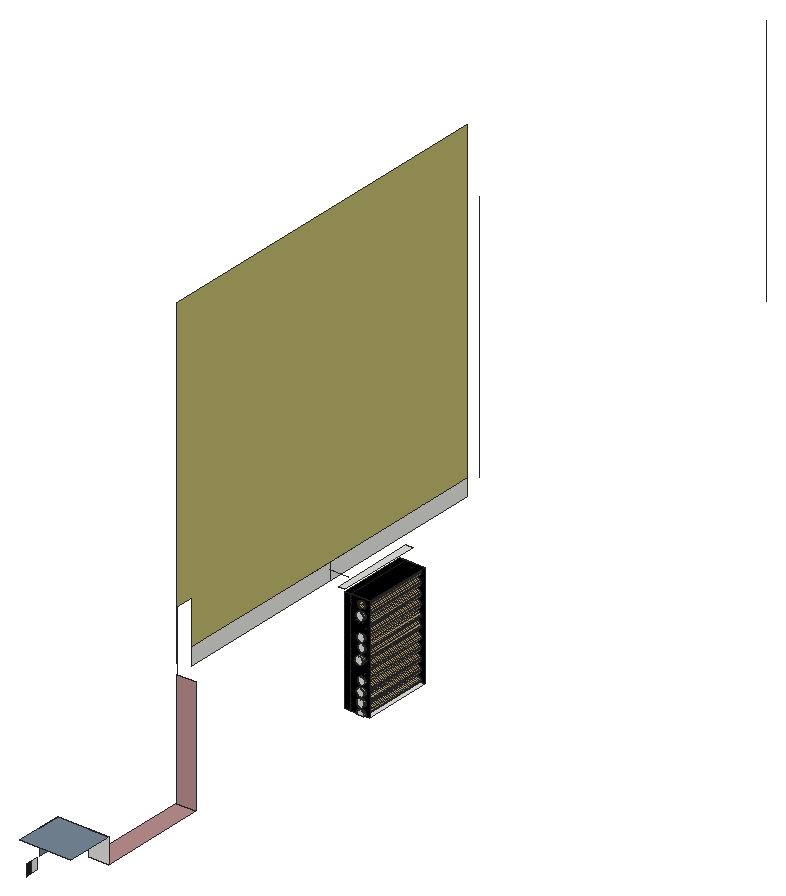
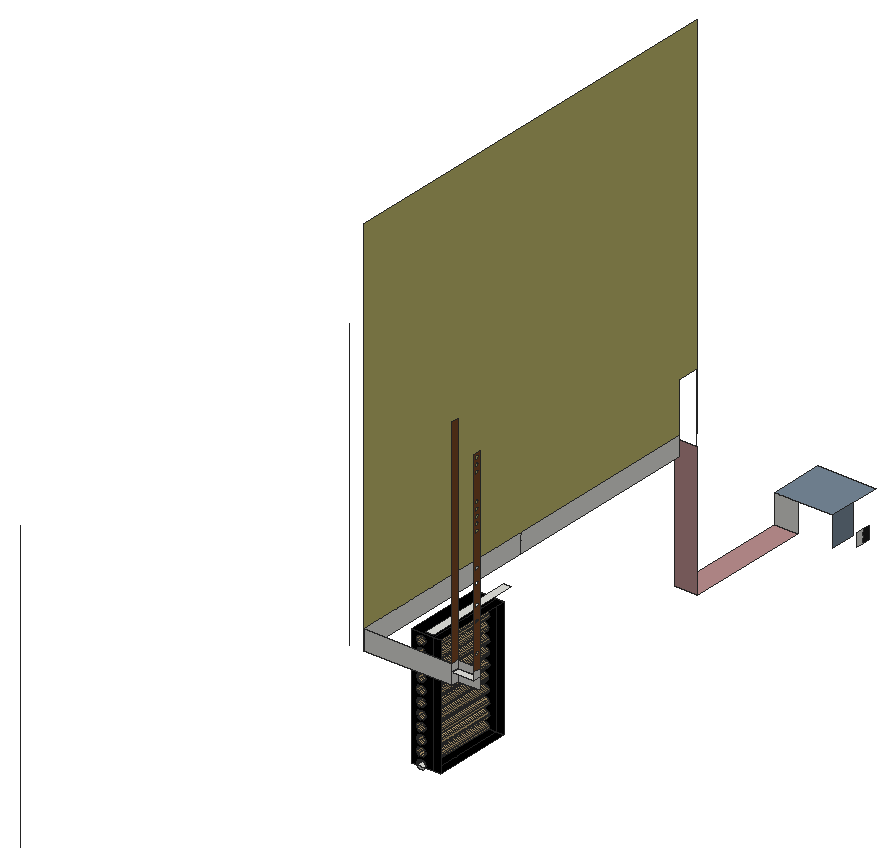
# SketchUp Ruby script. Lengths in inches.
U = 1.inch
M = Sketchup.active_model
def pt(a) = Geom::Point3d.new(a.map { |v| v * U })
def face(e, loops, mat)
  f = e.add_face(loops[0].map { |a| pt(a) })
  loops[1..].each { |l| e.add_face(l.map { |a| pt(a) }).erase! }
  f.material = f.back_material = mat if mat
  f
end
# faces: each face lists its corners as indices into pts; further lists are holes
def faces(e, pts, list, mat = nil) = list.each { |f| face(e, (f[0].is_a?(Array) ? f : [f]).map { |l| l.map { |i| pts[i] } }, mat) }
# xy, xz, yz: faces in a plane at the given z, y or x. An outline is a flat list of corners, or four numbers for a rectangle; further outlines are holes
def ring(l) = l.size == 4 ? [[l[0], l[1]], [l[2], l[1]], [l[2], l[3]], [l[0], l[3]]] : l.each_slice(2).to_a
def flat(e, list, mat, &to3) = list.each { |f| face(e, (f[0].is_a?(Array) ? f : [f]).map { |l| ring(l).map { |u, v| to3.(u, v) } }, mat) }
def xy(e, z, list, mat = nil) = flat(e, list, mat) { |x, y| [x, y, z] }
def xz(e, y, list, mat = nil) = flat(e, list, mat) { |x, z| [x, y, z] }
def yz(e, x, list, mat = nil) = flat(e, list, mat) { |y, z| [x, y, z] }
def lines(e, pts, list) = list.each { |a, b| e.add_line(pt(pts[a]), pt(pts[b])) }
# prism: a flat outline (further loops are holes) pulled along v
def prism(e, loops, v, mat = nil)
  f = face(e, loops, mat); d = Geom::Vector3d.new(v.map { |x| x * U })
  f.pushpull(f.normal.samedirection?(d) ? d.length : -d.length)
end
def box(e, o, s, mat = nil) = prism(e, [[o, [o[0] + s[0], o[1], o[2]], [o[0] + s[0], o[1] + s[1], o[2]], [o[0], o[1] + s[1], o[2]]]], [0, 0, s[2]], mat)
def at(x, y, z, deg = 0) = Geom::Transformation.translation(pt([x, y, z])) * Geom::Transformation.rotation(ORIGIN, Z_AXIS, deg.degrees)
def axes(o, x, y, z) = Geom::Transformation.new([*x, 0, *y, 0, *z, 0, *pt(o).to_a, 1])
def part(name) = M.definitions.add(name)
# library, detail: a bought-in or finely detailed component or shape, given as its bounding box
def library(name, o, s) = part(name).tap { |d| box(d.entities, o, s) }
def detail(e, o, s) = box(e.add_group.entities, o, s)
def put(e, d, t, mat = nil) = e.add_instance(d, t).tap { |i| i.material = mat if mat }
def group(e, t, mat = nil) = e.add_group.tap { |g| g.transformation = t; g.material = mat if mat }.entities
root = M.entities
M.materials.add("[0057_DarkKhaki]").color = [189, 183, 107]
M.materials.add("[0110_LightSlateGray]").color = [119, 136, 153]
M.materials.add("[0119_RosyBrown]").color = [188, 143, 143]
M.materials.add("[Color M08]").color = [30, 30, 30]
M.materials.add("[Color M09]").color = [0, 0, 0]
M.materials.add("[Wood Floor Light]").color = [204, 176, 127]
M.materials.add("[Wood Veneer 01]").color = [120, 70, 37]
xy(root,54.34,[[606.39,177.18,609.76,178.05],[606.39,178.05,609.76,210.93],[609.76,178.05,612,210.93]])
xy(root,54.34,[[600,178.05,603,210.93],[603,178.05,606.39,210.93]],"[Color M09]")
xy(root,60,[[602.49,22.38,612,74.42]],"[0119_RosyBrown]")
xy(root,72,[[587.78,0,612,22.38]],"[0110_LightSlateGray]")
xy(root,104.03,[[600,178.05,603,210.93],[603,178.05,612,210.93]],"[Color M09]")
xy(root,107.78,[[600,174.3,603,214.68]])
xy(root,120,[[557.23,244.17,566.2,247.17]])
xz(root,22.38,[[602.49,60,612,72]])
xz(root,74.42,[[602.73,120,603,144]])
xz(root,74.42,[[603,60,612,115.0625]],"[0119_RosyBrown]")
xz(root,176.24,[[608.08,76.28,608.55,76.34,608.98,76.52,609.36,76.81,609.65,77.1875,609.83,77.62,609.89,78.09,609.83,78.5625,609.65,79,609.36,79.375,608.98,79.66,608.55,79.84,608.08,79.9,607.61,79.84,607.17,79.66,606.79,79.375,606.51,79,606.33,78.5625,606.26,78.09,606.33,77.62,606.51,77.1875,606.79,76.81,607.17,76.52,607.61,76.34]])
xz(root,176.99,[[608.08,94.78,608.55,94.84,608.98,95.02,609.36,95.31,609.65,95.6875,609.83,96.12,609.89,96.59,609.83,97.0625,609.65,97.5,609.36,97.875,608.98,98.16,608.55,98.34,608.08,98.4,607.61,98.34,607.17,98.16,606.79,97.875,606.51,97.5,606.33,97.0625,606.26,96.59,606.33,96.12,606.51,95.6875,606.79,95.31,607.17,95.02,607.61,94.84]])
xz(root,177.05,[[608.08,62.4,608.55,62.47,608.98,62.65,609.36,62.94,609.65,63.3125,609.83,63.75,609.89,64.22,609.83,64.6875,609.65,65.125,609.36,65.5,608.98,65.79,608.55,65.97,608.08,66.03,607.61,65.97,607.17,65.79,606.79,65.5,606.51,65.125,606.33,64.6875,606.26,64.22,606.33,63.75,606.51,63.3125,606.79,62.94,607.17,62.65,607.61,62.47]])
xz(root,177.12,[[608.08,57.78,608.55,57.84,608.98,58.02,609.36,58.31,609.65,58.6875,609.83,59.12,609.89,59.59,609.83,60.0625,609.65,60.5,609.36,60.875,608.98,61.16,608.55,61.34,608.08,61.4,607.61,61.34,607.17,61.16,606.79,60.875,606.51,60.5,606.33,60.0625,606.26,59.59,606.33,59.12,606.51,58.6875,606.79,58.31,607.17,58.02,607.61,57.84]])
xz(root,177.18,[[606.39,54.34,609.76,54.34,609.83,54.5,609.89,54.97,609.83,55.4375,609.65,55.875,609.36,56.25,608.98,56.54,608.55,56.72,608.08,56.78,607.61,56.72,607.17,56.54,606.79,56.25,606.51,55.875,606.33,55.4375,606.26,54.97,606.33,54.5]])
xz(root,177.43,[[608.08,85.53,608.55,85.59,608.98,85.77,609.36,86.06,609.65,86.4375,609.83,86.87,609.89,87.34,609.83,87.8125,609.65,88.25,609.36,88.625,608.98,88.91,608.55,89.09,608.08,89.15,607.61,89.09,607.17,88.91,606.79,88.625,606.51,88.25,606.33,87.8125,606.26,87.34,606.33,86.87,606.51,86.4375,606.79,86.06,607.17,85.77,607.61,85.59]])
xz(root,177.8,[[608.08,67.03,608.55,67.09,608.98,67.27,609.36,67.56,609.65,67.9375,609.83,68.37,609.89,68.84,609.83,69.3125,609.65,69.75,609.36,70.125,608.98,70.41,608.55,70.59,608.08,70.65,607.61,70.59,607.17,70.41,606.79,70.125,606.51,69.75,606.33,69.3125,606.26,68.84,606.33,68.37,606.51,67.9375,606.79,67.56,607.17,67.27,607.61,67.09]])
xz(root,177.99,[[608.08,80.9,608.55,80.97,608.98,81.15,609.36,81.44,609.65,81.8125,609.83,82.25,609.89,82.72,609.83,83.1875,609.65,83.625,609.36,84,608.98,84.29,608.55,84.47,608.08,84.53,607.61,84.47,607.17,84.29,606.79,84,606.51,83.625,606.33,83.1875,606.26,82.72,606.33,82.25,606.51,81.8125,606.79,81.44,607.17,81.15,607.61,80.97]])
xz(root,178.05,[[600,54.34,603,104.03],[[603,54.34,612,104.03],[608.08,99.4,608.55,99.47,608.98,99.65,609.36,99.94,609.65,100.3125,609.83,100.75,609.89,101.22,609.83,101.6875,609.65,102.125,609.36,102.5,608.98,102.79,608.55,102.97,608.08,103.03,607.61,102.97,607.17,102.79,606.79,102.5,606.51,102.125,606.33,101.6875,606.26,101.22,606.33,100.75,606.51,100.3125,606.79,99.94,607.17,99.65,607.61,99.47]]],"[Color M09]")
xz(root,178.3,[[608.08,90.15,608.55,90.22,608.98,90.4,609.36,90.69,609.65,91.0625,609.83,91.5,609.89,91.97,609.83,92.4375,609.65,92.875,609.36,93.25,608.98,93.54,608.55,93.72,608.08,93.78,607.61,93.72,607.17,93.54,606.79,93.25,606.51,92.875,606.33,92.4375,606.26,91.97,606.33,91.5,606.51,91.0625,606.79,90.69,607.17,90.4,607.61,90.22]])
xz(root,178.37,[[608.08,71.65,608.55,71.72,608.98,71.9,609.36,72.19,609.65,72.5625,609.83,73,609.89,73.47,609.83,73.9375,609.65,74.375,609.36,74.75,608.98,75.04,608.55,75.22,608.08,75.28,607.61,75.22,607.17,75.04,606.79,74.75,606.51,74.375,606.33,73.9375,606.26,73.47,606.33,73,606.51,72.5625,606.79,72.19,607.17,71.9,607.61,71.72]])
xz(root,210.93,[[608.08,53.15,608.55,53.22,608.98,53.4,609.36,53.69,609.65,54.0625,609.76,54.34,606.39,54.34,606.51,54.0625,606.79,53.69,607.17,53.4,607.61,53.22]])
xz(root,210.93,[[600,54.34,603,104.03],[[603,54.34,606.39,54.34,606.33,54.5,606.26,54.97,606.33,55.4375,606.51,55.875,606.79,56.25,607.17,56.54,607.61,56.72,608.08,56.78,608.55,56.72,608.98,56.54,609.36,56.25,609.65,55.875,609.83,55.4375,609.89,54.97,609.83,54.5,609.76,54.34,612,54.34,612,104.03,603,104.03],[608.08,94.78,607.61,94.84,607.17,95.02,606.79,95.31,606.51,95.6875,606.33,96.12,606.26,96.59,606.33,97.0625,606.51,97.5,606.79,97.875,607.17,98.16,607.61,98.34,608.08,98.4,608.55,98.34,608.98,98.16,609.36,97.875,609.65,97.5,609.83,97.0625,609.89,96.59,609.83,96.12,609.65,95.6875,609.36,95.31,608.98,95.02,608.55,94.84],[608.08,90.15,607.61,90.22,607.17,90.4,606.79,90.69,606.51,91.0625,606.33,91.5,606.26,91.97,606.33,92.4375,606.51,92.875,606.79,93.25,607.17,93.54,607.61,93.72,608.08,93.78,608.55,93.72,608.98,93.54,609.36,93.25,609.65,92.875,609.83,92.4375,609.89,91.97,609.83,91.5,609.65,91.0625,609.36,90.69,608.98,90.4,608.55,90.22],[608.08,85.53,607.61,85.59,607.17,85.77,606.79,86.06,606.51,86.4375,606.33,86.87,606.26,87.34,606.33,87.8125,606.51,88.25,606.79,88.625,607.17,88.91,607.61,89.09,608.08,89.15,608.55,89.09,608.98,88.91,609.36,88.625,609.65,88.25,609.83,87.8125,609.89,87.34,609.83,86.87,609.65,86.4375,609.36,86.06,608.98,85.77,608.55,85.59],[608.08,80.9,607.61,80.97,607.17,81.15,606.79,81.44,606.51,81.8125,606.33,82.25,606.26,82.72,606.33,83.1875,606.51,83.625,606.79,84,607.17,84.29,607.61,84.47,608.08,84.53,608.55,84.47,608.98,84.29,609.36,84,609.65,83.625,609.83,83.1875,609.89,82.72,609.83,82.25,609.65,81.8125,609.36,81.44,608.98,81.15,608.55,80.97],[608.08,76.28,607.61,76.34,607.17,76.52,606.79,76.81,606.51,77.1875,606.33,77.62,606.26,78.09,606.33,78.5625,606.51,79,606.79,79.375,607.17,79.66,607.61,79.84,608.08,79.9,608.55,79.84,608.98,79.66,609.36,79.375,609.65,79,609.83,78.5625,609.89,78.09,609.83,77.62,609.65,77.1875,609.36,76.81,608.98,76.52,608.55,76.34],[608.08,71.65,607.61,71.72,607.17,71.9,606.79,72.19,606.51,72.5625,606.33,73,606.26,73.47,606.33,73.9375,606.51,74.375,606.79,74.75,607.17,75.04,607.61,75.22,608.08,75.28,608.55,75.22,608.98,75.04,609.36,74.75,609.65,74.375,609.83,73.9375,609.89,73.47,609.83,73,609.65,72.5625,609.36,72.19,608.98,71.9,608.55,71.72],[608.08,67.03,607.61,67.09,607.17,67.27,606.79,67.56,606.51,67.9375,606.33,68.37,606.26,68.84,606.33,69.3125,606.51,69.75,606.79,70.125,607.17,70.41,607.61,70.59,608.08,70.65,608.55,70.59,608.98,70.41,609.36,70.125,609.65,69.75,609.83,69.3125,609.89,68.84,609.83,68.37,609.65,67.9375,609.36,67.56,608.98,67.27,608.55,67.09],[608.08,62.4,607.61,62.47,607.17,62.65,606.79,62.94,606.51,63.3125,606.33,63.75,606.26,64.22,606.33,64.6875,606.51,65.125,606.79,65.5,607.17,65.79,607.61,65.97,608.08,66.03,608.55,65.97,608.98,65.79,609.36,65.5,609.65,65.125,609.83,64.6875,609.89,64.22,609.83,63.75,609.65,63.3125,609.36,62.94,608.98,62.65,608.55,62.47],[608.08,57.78,607.61,57.84,607.17,58.02,606.79,58.31,606.51,58.6875,606.33,59.12,606.26,59.59,606.33,60.0625,606.51,60.5,606.79,60.875,607.17,61.16,607.61,61.34,608.08,61.4,608.55,61.34,608.98,61.16,609.36,60.875,609.65,60.5,609.83,60.0625,609.89,59.59,609.83,59.12,609.65,58.6875,609.36,58.31,608.98,58.02,608.55,57.84],[608.08,99.4,607.61,99.47,607.17,99.65,606.79,99.94,606.51,100.3125,606.33,100.75,606.26,101.22,606.33,101.6875,606.51,102.125,606.79,102.5,607.17,102.79,607.61,102.97,608.08,103.03,608.55,102.97,608.98,102.79,609.36,102.5,609.65,102.125,609.83,101.6875,609.89,101.22,609.83,100.75,609.65,100.3125,609.36,99.94,608.98,99.65,608.55,99.47]]],"[Color M09]")
xz(root,244.17,[[557.23,115.0625,566.2,120],[557.23,120,566.2,123]])
xz(root,247.17,[[566.2,115.0625,603,123]])
yz(root,557.23,[[244.17,120,247.17,123]])
yz(root,557.23,[[[244.17,123,247.17,204],[245.69,201.45,245.94,201.48,246.16,201.58,246.36,201.73,246.5,201.92,246.6,202.15,246.63,202.39,246.6,202.63,246.5,202.86,246.36,203.05,246.16,203.2,245.94,203.29,245.69,203.33,245.45,203.29,245.22,203.2,245.03,203.05,244.88,202.86,244.79,202.63,244.75,202.39,244.79,202.15,244.88,201.92,245.03,201.73,245.22,201.58,245.45,201.48],[245.69,198.7,245.94,198.73,246.16,198.83,246.36,198.98,246.5,199.17,246.6,199.4,246.63,199.64,246.6,199.88,246.5,200.11,246.36,200.3,246.16,200.45,245.94,200.54,245.69,200.58,245.45,200.54,245.22,200.45,245.03,200.3,244.88,200.11,244.79,199.88,244.75,199.64,244.79,199.4,244.88,199.17,245.03,198.98,245.22,198.83,245.45,198.73],[245.69,195.95,245.94,195.98,246.16,196.08,246.36,196.23,246.5,196.42,246.6,196.65,246.63,196.89,246.6,197.13,246.5,197.36,246.36,197.55,246.16,197.7,245.94,197.79,245.69,197.83,245.45,197.79,245.22,197.7,245.03,197.55,244.88,197.36,244.79,197.13,244.75,196.89,244.79,196.65,244.88,196.42,245.03,196.23,245.22,196.08,245.45,195.98],[245.69,184.95,245.94,184.98,246.16,185.08,246.36,185.23,246.5,185.42,246.6,185.65,246.63,185.89,246.6,186.13,246.5,186.36,246.36,186.55,246.16,186.7,245.94,186.79,245.69,186.83,245.45,186.79,245.22,186.7,245.03,186.55,244.88,186.36,244.79,186.13,244.75,185.89,244.79,185.65,244.88,185.42,245.03,185.23,245.22,185.08,245.45,184.98],[245.69,182.2,245.94,182.23,246.16,182.33,246.36,182.48,246.5,182.67,246.6,182.9,246.63,183.14,246.6,183.38,246.5,183.61,246.36,183.8,246.16,183.95,245.94,184.04,245.69,184.08,245.45,184.04,245.22,183.95,245.03,183.8,244.88,183.61,244.79,183.38,244.75,183.14,244.79,182.9,244.88,182.67,245.03,182.48,245.22,182.33,245.45,182.23],[245.69,179.45,245.94,179.48,246.16,179.58,246.36,179.73,246.5,179.92,246.6,180.15,246.63,180.39,246.6,180.63,246.5,180.86,246.36,181.05,246.16,181.2,245.94,181.29,245.69,181.33,245.45,181.29,245.22,181.2,245.03,181.05,244.88,180.86,244.79,180.63,244.75,180.39,244.79,180.15,244.88,179.92,245.03,179.73,245.22,179.58,245.45,179.48],[245.69,176.7,245.94,176.73,246.16,176.83,246.36,176.98,246.5,177.17,246.6,177.4,246.63,177.64,246.6,177.88,246.5,178.11,246.36,178.3,246.16,178.45,245.94,178.54,245.69,178.58,245.45,178.54,245.22,178.45,245.03,178.3,244.88,178.11,244.79,177.88,244.75,177.64,244.79,177.4,244.88,177.17,245.03,176.98,245.22,176.83,245.45,176.73],[245.69,173.95,245.94,173.98,246.16,174.08,246.36,174.23,246.5,174.42,246.6,174.65,246.63,174.89,246.6,175.13,246.5,175.36,246.36,175.55,246.16,175.7,245.94,175.79,245.69,175.83,245.45,175.79,245.22,175.7,245.03,175.55,244.88,175.36,244.79,175.13,244.75,174.89,244.79,174.65,244.88,174.42,245.03,174.23,245.22,174.08,245.45,173.98],[245.69,160.2,245.94,160.23,246.16,160.33,246.36,160.48,246.5,160.67,246.6,160.9,246.63,161.14,246.6,161.38,246.5,161.61,246.36,161.8,246.16,161.95,245.94,162.04,245.69,162.08,245.45,162.04,245.22,161.95,245.03,161.8,244.88,161.61,244.79,161.38,244.75,161.14,244.79,160.9,244.88,160.67,245.03,160.48,245.22,160.33,245.45,160.23],[245.69,154.7,245.94,154.73,246.16,154.83,246.36,154.98,246.5,155.17,246.6,155.4,246.63,155.64,246.6,155.88,246.5,156.11,246.36,156.3,246.16,156.45,245.94,156.54,245.69,156.58,245.45,156.54,245.22,156.45,245.03,156.3,244.88,156.11,244.79,155.88,244.75,155.64,244.79,155.4,244.88,155.17,245.03,154.98,245.22,154.83,245.45,154.73],[245.69,146.45,245.94,146.48,246.16,146.58,246.36,146.73,246.5,146.92,246.6,147.15,246.63,147.39,246.6,147.63,246.5,147.86,246.36,148.05,246.16,148.2,245.94,148.29,245.69,148.33,245.45,148.29,245.22,148.2,245.03,148.05,244.88,147.86,244.79,147.63,244.75,147.39,244.79,147.15,244.88,146.92,245.03,146.73,245.22,146.58,245.45,146.48],[245.69,140.45,245.94,140.48,246.16,140.58,246.36,140.73,246.5,140.92,246.6,141.15,246.63,141.39,246.6,141.63,246.5,141.86,246.36,142.05,246.16,142.2,245.94,142.29,245.69,142.33,245.45,142.29,245.22,142.2,245.03,142.05,244.88,141.86,244.79,141.63,244.75,141.39,244.79,141.15,244.88,140.92,245.03,140.73,245.22,140.58,245.45,140.48],[245.69,128.45,245.94,128.48,246.16,128.58,246.36,128.73,246.5,128.92,246.6,129.15,246.63,129.39,246.6,129.63,246.5,129.86,246.36,130.05,246.16,130.2,245.94,130.29,245.69,130.33,245.45,130.29,245.22,130.2,245.03,130.05,244.88,129.86,244.79,129.63,244.75,129.39,244.79,129.15,244.88,128.92,245.03,128.73,245.22,128.58,245.45,128.48]]],"[Wood Veneer 01]")
yz(root,566.2,[[244.17,115.0625,247.17,120],[244.17,120,247.17,123]])
yz(root,566.2,[[244.17,123,247.17,212.97]],"[Wood Veneer 01]")
yz(root,587.78,[[6.88,54.6875,9.88,60]])
yz(root,587.78,[[12,60,22.38,72]],"[0110_LightSlateGray]")
yz(root,587.78,[[3.88,54.6875,6.88,60]],"[Color M08]")
yz(root,603,[[83.42,115.0625,165.3,123],[165.3,115.0625,247.17,123]])
yz(root,603,[[83.42,123,83.42,144,74.42,144,74.42,273.75,247.17,273.75,247.17,123]],"[0057_DarkKhaki]")
p = [[606.33,210.93,54.5],[606.39,210.93,54.34],[606.39,178.05,54.34],[606.39,177.18,54.34],[606.33,177.18,54.5],[609.76,210.93,54.34],
  [609.83,210.93,54.5],[609.83,177.18,54.5],[609.76,177.18,54.34],[609.76,178.05,54.34],[606.26,210.93,54.97],[606.26,177.18,54.97],
  [609.89,210.93,54.97],[609.89,177.18,54.97],[606.33,210.93,55.4375],[606.33,177.18,55.4375],[609.83,210.93,55.4375],[609.83,177.18,55.4375],
  [606.51,210.93,55.875],[606.51,177.18,55.875],[609.65,210.93,55.875],[609.65,177.18,55.875],[606.79,210.93,56.25],[606.79,177.18,56.25],
  [609.36,210.93,56.25],[609.36,177.18,56.25],[607.17,210.93,56.54],[607.17,177.18,56.54],[608.98,210.93,56.54],[608.98,177.18,56.54],
  [607.61,210.93,56.72],[607.61,177.18,56.72],[608.55,210.93,56.72],[608.55,177.18,56.72],[608.08,210.93,56.78],[608.08,177.18,56.78],
  [607.17,210.93,58.02],[607.61,210.93,57.84],[607.61,177.12,57.84],[607.17,177.12,58.02],[608.08,210.93,57.78],[608.08,177.12,57.78],
  [608.55,210.93,57.84],[608.55,177.12,57.84],[608.98,210.93,58.02],[608.98,177.12,58.02],[606.79,210.93,58.31],[606.79,177.12,58.31],
  [609.36,210.93,58.31],[609.36,177.12,58.31],[606.51,210.93,58.6875],[606.51,177.12,58.6875],[609.65,210.93,58.6875],[609.65,177.12,58.6875],
  [606.33,210.93,59.12],[606.33,177.12,59.12],[609.83,210.93,59.12],[609.83,177.12,59.12],[606.26,210.93,59.59],[606.26,177.12,59.59],
  [609.89,210.93,59.59],[609.89,177.12,59.59],[606.33,210.93,60.0625],[606.33,177.12,60.0625],[609.83,210.93,60.0625],[609.83,177.12,60.0625],
  [606.51,210.93,60.5],[606.51,177.12,60.5],[609.65,210.93,60.5],[609.65,177.12,60.5],[606.79,210.93,60.875],[606.79,177.12,60.875],
  [609.36,210.93,60.875],[609.36,177.12,60.875],[607.17,210.93,61.16],[607.17,177.12,61.16],[608.98,210.93,61.16],[608.98,177.12,61.16],
  [607.61,210.93,61.34],[607.61,177.12,61.34],[608.55,210.93,61.34],[608.55,177.12,61.34],[608.08,210.93,61.4],[608.08,177.12,61.4],
  [607.61,210.93,62.47],[608.08,210.93,62.4],[608.08,177.05,62.4],[607.61,177.05,62.47],[608.55,210.93,62.47],[608.55,177.05,62.47],
  [607.17,210.93,62.65],[607.17,177.05,62.65],[608.98,210.93,62.65],[608.98,177.05,62.65],[606.79,210.93,62.94],[606.79,177.05,62.94],
  [609.36,210.93,62.94],[609.36,177.05,62.94],[606.51,210.93,63.3125],[606.51,177.05,63.3125],[609.65,210.93,63.3125],[609.65,177.05,63.3125],
  [606.33,210.93,63.75],[606.33,177.05,63.75],[609.83,210.93,63.75],[609.83,177.05,63.75],[606.26,210.93,64.22],[606.26,177.05,64.22],
  [609.89,210.93,64.22],[609.89,177.05,64.22],[606.33,210.93,64.6875],[606.33,177.05,64.6875],[609.83,210.93,64.6875],[609.83,177.05,64.6875],
  [606.51,210.93,65.125],[606.51,177.05,65.125],[609.65,210.93,65.125],[609.65,177.05,65.125],[606.79,210.93,65.5],[606.79,177.05,65.5],
  [609.36,210.93,65.5],[609.36,177.05,65.5],[607.17,210.93,65.79],[607.17,177.05,65.79],[608.98,210.93,65.79],[608.98,177.05,65.79],
  [607.61,210.93,65.97],[607.61,177.05,65.97],[608.55,210.93,65.97],[608.55,177.05,65.97],[608.08,210.93,66.03],[608.08,177.05,66.03],
  [607.61,210.93,67.09],[608.08,210.93,67.03],[608.08,177.8,67.03],[607.61,177.8,67.09],[608.55,210.93,67.09],[608.55,177.8,67.09],
  [607.17,210.93,67.27],[607.17,177.8,67.27],[608.98,210.93,67.27],[608.98,177.8,67.27],[606.79,210.93,67.56],[606.79,177.8,67.56],
  [609.36,210.93,67.56],[609.36,177.8,67.56],[606.51,210.93,67.9375],[606.51,177.8,67.9375],[609.65,210.93,67.9375],[609.65,177.8,67.9375],
  [606.33,210.93,68.37],[606.33,177.8,68.37],[609.83,210.93,68.37],[609.83,177.8,68.37],[606.26,210.93,68.84],[606.26,177.8,68.84],
  [609.89,210.93,68.84],[609.89,177.8,68.84],[606.33,210.93,69.3125],[606.33,177.8,69.3125],[609.83,210.93,69.3125],[609.83,177.8,69.3125],
  [606.51,210.93,69.75],[606.51,177.8,69.75],[609.65,210.93,69.75],[609.65,177.8,69.75],[606.79,210.93,70.125],[606.79,177.8,70.125],
  [609.36,210.93,70.125],[609.36,177.8,70.125],[607.17,210.93,70.41],[607.17,177.8,70.41],[608.98,210.93,70.41],[608.98,177.8,70.41],
  [607.61,210.93,70.59],[607.61,177.8,70.59],[608.55,210.93,70.59],[608.55,177.8,70.59],[608.08,210.93,70.65],[608.08,177.8,70.65],
  [607.17,210.93,71.9],[607.61,210.93,71.72],[607.61,178.37,71.72],[607.17,178.37,71.9],[608.08,210.93,71.65],[608.08,178.37,71.65],
  [608.55,210.93,71.72],[608.55,178.37,71.72],[608.98,210.93,71.9],[608.98,178.37,71.9],[606.79,210.93,72.19],[606.79,178.37,72.19],
  [609.36,210.93,72.19],[609.36,178.37,72.19],[606.51,210.93,72.5625],[606.51,178.37,72.5625],[609.65,210.93,72.5625],[609.65,178.37,72.5625],
  [606.33,210.93,73],[606.33,178.37,73],[609.83,210.93,73],[609.83,178.37,73],[606.26,210.93,73.47],[606.26,178.37,73.47],
  [609.89,210.93,73.47],[609.89,178.37,73.47],[606.33,210.93,73.9375],[606.33,178.37,73.9375],[609.83,210.93,73.9375],[609.83,178.37,73.9375],
  [606.51,210.93,74.375],[606.51,178.37,74.375],[609.65,210.93,74.375],[609.65,178.37,74.375],[606.79,210.93,74.75],[606.79,178.37,74.75],
  [609.36,210.93,74.75],[609.36,178.37,74.75],[607.17,210.93,75.04],[607.17,178.37,75.04],[608.98,210.93,75.04],[608.98,178.37,75.04],
  [607.61,210.93,75.22],[607.61,178.37,75.22],[608.55,210.93,75.22],[608.55,178.37,75.22],[608.08,210.93,75.28],[608.08,178.37,75.28],
  [607.17,210.93,76.52],[607.61,210.93,76.34],[607.61,176.24,76.34],[607.17,176.24,76.52],[608.08,210.93,76.28],[608.08,176.24,76.28],
  [608.55,210.93,76.34],[608.55,176.24,76.34],[608.98,210.93,76.52],[608.98,176.24,76.52],[606.79,210.93,76.81],[606.79,176.24,76.81],
  [609.36,210.93,76.81],[609.36,176.24,76.81],[606.51,210.93,77.1875],[606.51,176.24,77.1875],[609.65,210.93,77.1875],[609.65,176.24,77.1875],
  [606.33,210.93,77.62],[606.33,176.24,77.62],[609.83,210.93,77.62],[609.83,176.24,77.62],[606.26,210.93,78.09],[606.26,176.24,78.09],
  [609.89,210.93,78.09],[609.89,176.24,78.09],[606.33,210.93,78.5625],[606.33,176.24,78.5625],[609.83,210.93,78.5625],[609.83,176.24,78.5625],
  [606.51,210.93,79],[606.51,176.24,79],[609.65,210.93,79],[609.65,176.24,79],[606.79,210.93,79.375],[606.79,176.24,79.375],
  [609.36,210.93,79.375],[609.36,176.24,79.375],[607.17,210.93,79.66],[607.17,176.24,79.66],[608.98,210.93,79.66],[608.98,176.24,79.66],
  [607.61,210.93,79.84],[607.61,176.24,79.84],[608.55,210.93,79.84],[608.55,176.24,79.84],[608.08,210.93,79.9],[608.08,176.24,79.9],
  [607.61,210.93,80.97],[608.08,210.93,80.9],[608.08,177.99,80.9],[607.61,177.99,80.97],[608.55,210.93,80.97],[608.55,177.99,80.97],
  [607.17,210.93,81.15],[607.17,177.99,81.15],[608.98,210.93,81.15],[608.98,177.99,81.15],[606.79,210.93,81.44],[606.79,177.99,81.44],
  [609.36,210.93,81.44],[609.36,177.99,81.44],[606.51,210.93,81.8125],[606.51,177.99,81.8125],[609.65,210.93,81.8125],[609.65,177.99,81.8125],
  [606.33,210.93,82.25],[606.33,177.99,82.25],[609.83,210.93,82.25],[609.83,177.99,82.25],[606.26,210.93,82.72],[606.26,177.99,82.72],
  [609.89,210.93,82.72],[609.89,177.99,82.72],[606.33,210.93,83.1875],[606.33,177.99,83.1875],[609.83,210.93,83.1875],[609.83,177.99,83.1875],
  [606.51,210.93,83.625],[606.51,177.99,83.625],[609.65,210.93,83.625],[609.65,177.99,83.625],[606.79,210.93,84],[606.79,177.99,84],
  [609.36,210.93,84],[609.36,177.99,84],[607.17,210.93,84.29],[607.17,177.99,84.29],[608.98,210.93,84.29],[608.98,177.99,84.29],
  [607.61,210.93,84.47],[607.61,177.99,84.47],[608.55,210.93,84.47],[608.55,177.99,84.47],[608.08,210.93,84.53],[608.08,177.99,84.53],
  [607.61,210.93,85.59],[608.08,210.93,85.53],[608.08,177.43,85.53],[607.61,177.43,85.59],[608.55,210.93,85.59],[608.55,177.43,85.59],
  [607.17,210.93,85.77],[607.17,177.43,85.77],[608.98,210.93,85.77],[608.98,177.43,85.77],[606.79,210.93,86.06],[606.79,177.43,86.06],
  [609.36,210.93,86.06],[609.36,177.43,86.06],[606.51,210.93,86.4375],[606.51,177.43,86.4375],[609.65,210.93,86.4375],[609.65,177.43,86.4375],
  [606.33,210.93,86.87],[606.33,177.43,86.87],[609.83,210.93,86.87],[609.83,177.43,86.87],[606.26,210.93,87.34],[606.26,177.43,87.34],
  [609.89,210.93,87.34],[609.89,177.43,87.34],[606.33,210.93,87.8125],[606.33,177.43,87.8125],[609.83,210.93,87.8125],[609.83,177.43,87.8125],
  [606.51,210.93,88.25],[606.51,177.43,88.25],[609.65,210.93,88.25],[609.65,177.43,88.25],[606.79,210.93,88.625],[606.79,177.43,88.625],
  [609.36,210.93,88.625],[609.36,177.43,88.625],[607.17,210.93,88.91],[607.17,177.43,88.91],[608.98,210.93,88.91],[608.98,177.43,88.91],
  [607.61,210.93,89.09],[607.61,177.43,89.09],[608.55,210.93,89.09],[608.55,177.43,89.09],[608.08,210.93,89.15],[608.08,177.43,89.15],
  [607.17,210.93,90.4],[607.61,210.93,90.22],[607.61,178.3,90.22],[607.17,178.3,90.4],[608.08,210.93,90.15],[608.08,178.3,90.15],
  [608.55,210.93,90.22],[608.55,178.3,90.22],[608.98,210.93,90.4],[608.98,178.3,90.4],[606.79,210.93,90.69],[606.79,178.3,90.69],
  [609.36,210.93,90.69],[609.36,178.3,90.69],[606.51,210.93,91.0625],[606.51,178.3,91.0625],[609.65,210.93,91.0625],[609.65,178.3,91.0625],
  [606.33,210.93,91.5],[606.33,178.3,91.5],[609.83,210.93,91.5],[609.83,178.3,91.5],[606.26,210.93,91.97],[606.26,178.3,91.97],
  [609.89,210.93,91.97],[609.89,178.3,91.97],[606.33,210.93,92.4375],[606.33,178.3,92.4375],[609.83,210.93,92.4375],[609.83,178.3,92.4375],
  [606.51,210.93,92.875],[606.51,178.3,92.875],[609.65,210.93,92.875],[609.65,178.3,92.875],[606.79,210.93,93.25],[606.79,178.3,93.25],
  [609.36,210.93,93.25],[609.36,178.3,93.25],[607.17,210.93,93.54],[607.17,178.3,93.54],[608.98,210.93,93.54],[608.98,178.3,93.54],
  [607.61,210.93,93.72],[607.61,178.3,93.72],[608.55,210.93,93.72],[608.55,178.3,93.72],[608.08,210.93,93.78],[608.08,178.3,93.78],
  [607.17,210.93,95.02],[607.61,210.93,94.84],[607.61,176.99,94.84],[607.17,176.99,95.02],[608.08,210.93,94.78],[608.08,176.99,94.78],
  [608.55,210.93,94.84],[608.55,176.99,94.84],[608.98,210.93,95.02],[608.98,176.99,95.02],[606.79,210.93,95.31],[606.79,176.99,95.31],
  [609.36,210.93,95.31],[609.36,176.99,95.31],[606.51,210.93,95.6875],[606.51,176.99,95.6875],[609.65,210.93,95.6875],[609.65,176.99,95.6875],
  [606.33,210.93,96.12],[606.33,176.99,96.12],[609.83,210.93,96.12],[609.83,176.99,96.12],[606.26,210.93,96.59],[606.26,176.99,96.59],
  [609.89,210.93,96.59],[609.89,176.99,96.59],[606.33,210.93,97.0625],[606.33,176.99,97.0625],[609.83,210.93,97.0625],[609.83,176.99,97.0625],
  [606.51,210.93,97.5],[606.51,176.99,97.5],[609.65,210.93,97.5],[609.65,176.99,97.5],[606.79,210.93,97.875],[606.79,176.99,97.875],
  [609.36,210.93,97.875],[609.36,176.99,97.875],[607.17,210.93,98.16],[607.17,176.99,98.16],[608.98,210.93,98.16],[608.98,176.99,98.16],
  [607.61,210.93,98.34],[607.61,176.99,98.34],[608.55,210.93,98.34],[608.55,176.99,98.34],[608.08,210.93,98.4],[608.08,176.99,98.4],
  [607.61,210.93,99.47],[608.08,210.93,99.4],[608.08,178.05,99.4],[607.61,178.05,99.47],[608.55,210.93,99.47],[608.55,178.05,99.47],
  [607.17,210.93,99.65],[607.17,178.05,99.65],[608.98,210.93,99.65],[608.98,178.05,99.65],[606.79,210.93,99.94],[606.79,178.05,99.94],
  [609.36,210.93,99.94],[609.36,178.05,99.94],[606.51,210.93,100.3125],[606.51,178.05,100.3125],[609.65,210.93,100.3125],[609.65,178.05,100.3125],
  [606.33,210.93,100.75],[606.33,178.05,100.75],[609.83,210.93,100.75],[609.83,178.05,100.75],[606.26,210.93,101.22],[606.26,178.05,101.22],
  [609.89,210.93,101.22],[609.89,178.05,101.22],[606.33,210.93,101.6875],[606.33,178.05,101.6875],[609.83,210.93,101.6875],[609.83,178.05,101.6875],
  [606.51,210.93,102.125],[606.51,178.05,102.125],[609.65,210.93,102.125],[609.65,178.05,102.125],[606.79,210.93,102.5],[606.79,178.05,102.5],
  [609.36,210.93,102.5],[609.36,178.05,102.5],[607.17,210.93,102.79],[607.17,178.05,102.79],[608.98,210.93,102.79],[608.98,178.05,102.79],
  [607.61,210.93,102.97],[607.61,178.05,102.97],[608.55,210.93,102.97],[608.55,178.05,102.97],[608.08,210.93,103.03],[608.08,178.05,103.03],
  [603,254.42,120],[603,254.42,240],[603,425.42,120],[603,425.42,240],[603,165.3,120],[612,165.3,120],
  [603,74.42,120],[603,74.42,115.0625]]
faces(root,p,[[0,1,2,3,4],[5,6,7,8,9],[10,0,4,11],[6,12,13,7],[14,10,11,15],[12,16,17,13],[18,14,15,19],[16,20,21,17],
  [22,18,19,23],[20,24,25,21],[26,22,23,27],[24,28,29,25],[30,26,27,31],[28,32,33,29],[34,30,31,35],[32,34,35,33],
  [36,37,38,39],[37,40,41,38],[40,42,43,41],[42,44,45,43],[46,36,39,47],[44,48,49,45],[50,46,47,51],[48,52,53,49],
  [54,50,51,55],[52,56,57,53],[58,54,55,59],[56,60,61,57],[62,58,59,63],[60,64,65,61],[66,62,63,67],[64,68,69,65],
  [70,66,67,71],[68,72,73,69],[74,70,71,75],[72,76,77,73],[78,74,75,79],[76,80,81,77],[82,78,79,83],[80,82,83,81],
  [84,85,86,87],[85,88,89,86],[90,84,87,91],[88,92,93,89],[94,90,91,95],[92,96,97,93],[98,94,95,99],[96,100,101,97],
  [102,98,99,103],[100,104,105,101],[106,102,103,107],[104,108,109,105],[110,106,107,111],[108,112,113,109],[114,110,111,115],[112,116,117,113],
  [118,114,115,119],[116,120,121,117],[122,118,119,123],[120,124,125,121],[126,122,123,127],[124,128,129,125],[130,126,127,131],[128,130,131,129],
  [132,133,134,135],[133,136,137,134],[138,132,135,139],[136,140,141,137],[142,138,139,143],[140,144,145,141],[146,142,143,147],[144,148,149,145],
  [150,146,147,151],[148,152,153,149],[154,150,151,155],[152,156,157,153],[158,154,155,159],[156,160,161,157],[162,158,159,163],[160,164,165,161],
  [166,162,163,167],[164,168,169,165],[170,166,167,171],[168,172,173,169],[174,170,171,175],[172,176,177,173],[178,174,175,179],[176,178,179,177],
  [180,181,182,183],[181,184,185,182],[184,186,187,185],[186,188,189,187],[190,180,183,191],[188,192,193,189],[194,190,191,195],[192,196,197,193],
  [198,194,195,199],[196,200,201,197],[202,198,199,203],[200,204,205,201],[206,202,203,207],[204,208,209,205],[210,206,207,211],[208,212,213,209],
  [214,210,211,215],[212,216,217,213],[218,214,215,219],[216,220,221,217],[222,218,219,223],[220,224,225,221],[226,222,223,227],[224,226,227,225],
  [228,229,230,231],[229,232,233,230],[232,234,235,233],[234,236,237,235],[238,228,231,239],[236,240,241,237],[242,238,239,243],[240,244,245,241],
  [246,242,243,247],[244,248,249,245],[250,246,247,251],[248,252,253,249],[254,250,251,255],[252,256,257,253],[258,254,255,259],[256,260,261,257],
  [262,258,259,263],[260,264,265,261],[266,262,263,267],[264,268,269,265],[270,266,267,271],[268,272,273,269],[274,270,271,275],[272,274,275,273],
  [276,277,278,279],[277,280,281,278],[282,276,279,283],[280,284,285,281],[286,282,283,287],[284,288,289,285],[290,286,287,291],[288,292,293,289],
  [294,290,291,295],[292,296,297,293],[298,294,295,299],[296,300,301,297],[302,298,299,303],[300,304,305,301],[306,302,303,307],[304,308,309,305],
  [310,306,307,311],[308,312,313,309],[314,310,311,315],[312,316,317,313],[318,314,315,319],[316,320,321,317],[322,318,319,323],[320,322,323,321],
  [324,325,326,327],[325,328,329,326],[330,324,327,331],[328,332,333,329],[334,330,331,335],[332,336,337,333],[338,334,335,339],[336,340,341,337],
  [342,338,339,343],[340,344,345,341],[346,342,343,347],[344,348,349,345],[350,346,347,351],[348,352,353,349],[354,350,351,355],[352,356,357,353],
  [358,354,355,359],[356,360,361,357],[362,358,359,363],[360,364,365,361],[366,362,363,367],[364,368,369,365],[370,366,367,371],[368,370,371,369],
  [372,373,374,375],[373,376,377,374],[376,378,379,377],[378,380,381,379],[382,372,375,383],[380,384,385,381],[386,382,383,387],[384,388,389,385],
  [390,386,387,391],[388,392,393,389],[394,390,391,395],[392,396,397,393],[398,394,395,399],[396,400,401,397],[402,398,399,403],[400,404,405,401],
  [406,402,403,407],[404,408,409,405],[410,406,407,411],[408,412,413,409],[414,410,411,415],[412,416,417,413],[418,414,415,419],[416,418,419,417],
  [420,421,422,423],[421,424,425,422],[424,426,427,425],[426,428,429,427],[430,420,423,431],[428,432,433,429],[434,430,431,435],[432,436,437,433],
  [438,434,435,439],[436,440,441,437],[442,438,439,443],[440,444,445,441],[446,442,443,447],[444,448,449,445],[450,446,447,451],[448,452,453,449],
  [454,450,451,455],[452,456,457,453],[458,454,455,459],[456,460,461,457],[462,458,459,463],[460,464,465,461],[466,462,463,467],[464,466,467,465],
  [468,469,470,471],[469,472,473,470],[474,468,471,475],[472,476,477,473],[478,474,475,479],[476,480,481,477],[482,478,479,483],[480,484,485,481],
  [486,482,483,487],[484,488,489,485],[490,486,487,491],[488,492,493,489],[494,490,491,495],[492,496,497,493],[498,494,495,499],[496,500,501,497],
  [502,498,499,503],[500,504,505,501],[506,502,503,507],[504,508,509,505],[510,506,507,511],[508,512,513,509],[514,510,511,515],[512,514,515,513]],"[Wood Floor Light]")
lines(root,p,[[516,517],[518,519],[520,521],[522,523]])
